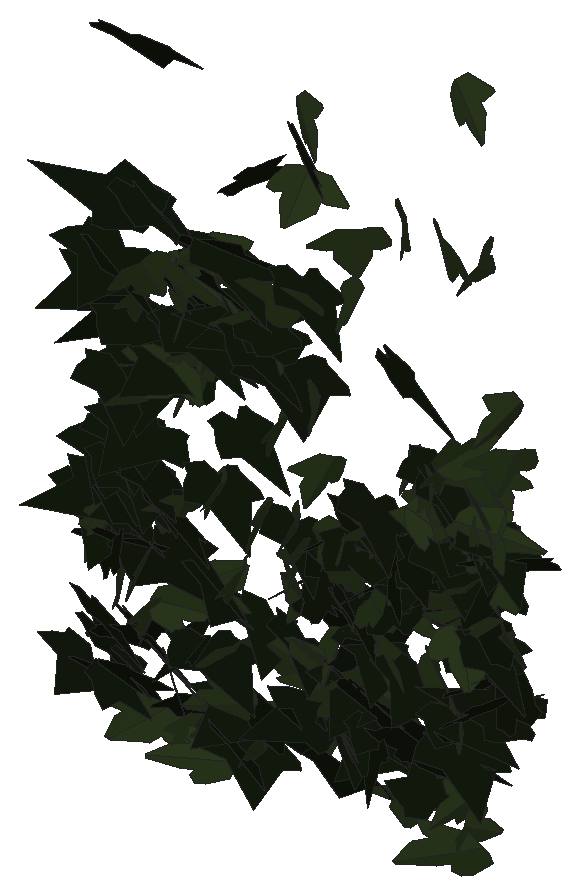
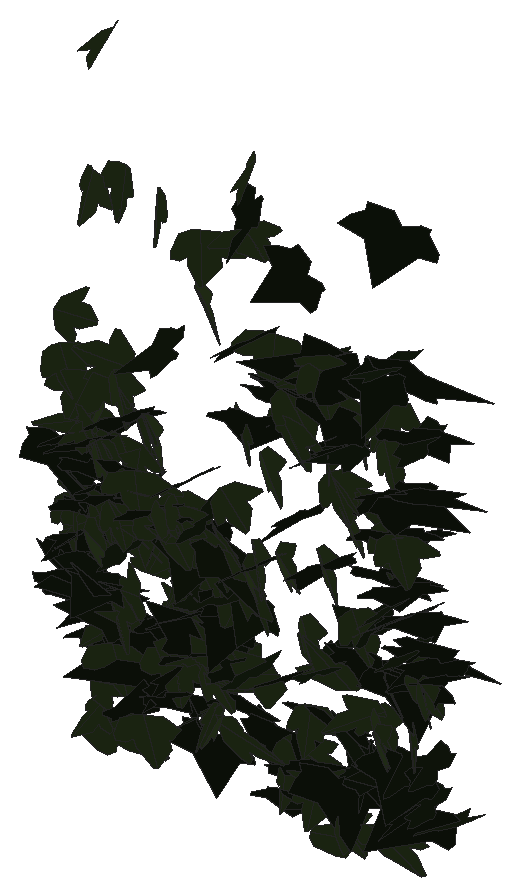
# SketchUp Ruby script. Lengths in millimetres.
U = 1.mm
M = Sketchup.active_model
def pt(a) = Geom::Point3d.new(a.map { |v| v * U })
def face(e, loops, mat)
  f = e.add_face(loops[0].map { |a| pt(a) })
  loops[1..].each { |l| e.add_face(l.map { |a| pt(a) }).erase! }
  f.material = f.back_material = mat if mat
  f
end
# faces: each face lists its corners as indices into pts; further lists are holes
def faces(e, pts, list, mat = nil) = list.each { |f| face(e, (f[0].is_a?(Array) ? f : [f]).map { |l| l.map { |i| pts[i] } }, mat) }
# xy, xz, yz: faces in a plane at the given z, y or x. An outline is a flat list of corners, or four numbers for a rectangle; further outlines are holes
def ring(l) = l.size == 4 ? [[l[0], l[1]], [l[2], l[1]], [l[2], l[3]], [l[0], l[3]]] : l.each_slice(2).to_a
def flat(e, list, mat, &to3) = list.each { |f| face(e, (f[0].is_a?(Array) ? f : [f]).map { |l| ring(l).map { |u, v| to3.(u, v) } }, mat) }
def xy(e, z, list, mat = nil) = flat(e, list, mat) { |x, y| [x, y, z] }
def xz(e, y, list, mat = nil) = flat(e, list, mat) { |x, z| [x, y, z] }
def yz(e, x, list, mat = nil) = flat(e, list, mat) { |y, z| [x, y, z] }
def lines(e, pts, list) = list.each { |a, b| e.add_line(pt(pts[a]), pt(pts[b])) }
# prism: a flat outline (further loops are holes) pulled along v
def prism(e, loops, v, mat = nil)
  f = face(e, loops, mat); d = Geom::Vector3d.new(v.map { |x| x * U })
  f.pushpull(f.normal.samedirection?(d) ? d.length : -d.length)
end
def box(e, o, s, mat = nil) = prism(e, [[o, [o[0] + s[0], o[1], o[2]], [o[0] + s[0], o[1] + s[1], o[2]], [o[0], o[1] + s[1], o[2]]]], [0, 0, s[2]], mat)
def at(x, y, z, deg = 0) = Geom::Transformation.translation(pt([x, y, z])) * Geom::Transformation.rotation(ORIGIN, Z_AXIS, deg.degrees)
def axes(o, x, y, z) = Geom::Transformation.new([*x, 0, *y, 0, *z, 0, *pt(o).to_a, 1])
def part(name) = M.definitions.add(name)
# library, detail: a bought-in or finely detailed component or shape, given as its bounding box
def library(name, o, s) = part(name).tap { |d| box(d.entities, o, s) }
def detail(e, o, s) = box(e.add_group.entities, o, s)
def put(e, d, t, mat = nil) = e.add_instance(d, t).tap { |i| i.material = mat if mat }
def group(e, t, mat = nil) = e.add_group.tap { |g| g.transformation = t; g.material = mat if mat }.entities
root = M.entities
M.materials.add("efeu1").color = [18, 25, 13]
M.materials.add("efeu2").color = [43, 57, 29]
c1 = part("ivyleaf_9")
p = [[39.1,54.8,31.7],[34.5,51.8,30.2],[-5.3,25.2,17.3],[-17.9,28.3,20.9],[-21.6,21.7,17],[-20.2,4.3,5.3],
  [-22.9,-0.3,2.5],[-17.1,-4,-0.6],[-2,-2.1,-1.2],[-0.7,-15.4,-10.1],[16.6,-22.3,-16.7],[21.1,-15.1,-12.5],
  [32.7,-10.7,-11],[46.1,-1.8,-6.6],[30.8,11.2,3.8]]
faces(c1.entities,p,[[0,1,2,3,4,5,6,7,8,9,10,11,12,13,14]],"efeu1")
c2 = part("ivyleaf_10")
p = [[0,12.8,-0.8],[-1.5,51.3,-10.9],[-4.9,51,-11.6],[-13.6,26.5,-7.3],[-13.2,15.9,-4.6],[-21.1,19.3,-7.2],
  [-29.5,16.3,-8.3],[-29.2,8.3,-6.2],[-19.7,-9.8,0.5],[-7.6,-13,4],[1,-12.2,5.8],[-0.4,51.1,-11.1],
  [-1.5,51.1,-10.9],[1,-12.4,5.9],[16.9,-12.4,3.5],[35.1,9.1,-5.1],[35,12.9,-6.1],[20.5,16.4,-4.9],
  [15.8,15,-3.8],[15.3,27.6,-7.1],[12.8,31.3,-7.8]]
faces(c2.entities,p,[[0,1,2,3,4,5,6,7,8,9,10],[11,12,0,13,14,15,16,17,18,19,20]],"efeu2")
put(root,c1,axes([2557.7,915.6,1679.3],[-0.86235,-0.55381,0.54649],[-0.10783,-0.60725,-0.66235],[1.47685,-0.36771,0.27074]))
put(root,c1,axes([2578.8,934.3,2103.4],[-1.36513,-0.35723,0.44081],[-0.65601,-0.29003,-0.79592],[0.85774,-0.79037,0.09283]))
put(root,c1,axes([2557.4,913.3,1886.7],[0.10613,-0.67564,-0.60536],[0.2115,0.60703,-0.66726],[1.71352,-0.03308,0.11986]))
put(root,c2,axes([2575.1,914.1,1848.5],[0.08886,-0.79996,0.47142],[0.28061,-0.45964,-0.79457],[1.74477,0.11466,0.10378]))
put(root,c1,axes([2606.9,906.4,1885.8],[-1.54143,-0.14502,0.48085],[-0.90155,-0.08261,-0.82279],[0.31763,-0.93827,-0.00187]))
put(root,c1,axes([2557.1,925.3,1711.7],[0.82056,-0.74571,0.10087],[0.11253,-0.08233,-0.86132],[1.42774,0.43507,0.00991]))
put(root,c1,axes([2581.2,918.6,1856.9],[-0.7542,-0.79037,0.17718],[-0.09998,-0.17176,-0.88366],[1.53833,-0.39866,0.02944]))
put(root,c2,axes([2589.2,911.8,1862.9],[-0.09793,-0.72878,0.5131],[0.07641,-0.51532,-0.72791],[1.69456,-0.01888,0.06247]))
put(root,c1,axes([2603.4,926.1,2086.3],[-0.25433,0.15373,-0.90287],[0.02132,-0.91209,-0.15696],[-1.74294,-0.03359,0.12983]))
put(root,c1,axes([2626.3,899.9,2221],[-0.73213,0.23685,0.83177],[-1.52357,0.24695,-0.44056],[-0.62282,-0.88252,0.09995]))
put(root,c1,axes([2565.3,910.4,1748],[0.6819,-0.74519,0.28542],[0.26081,-0.25077,-0.82673],[1.49616,0.38335,0.01403]))
put(root,c1,axes([2592.5,919.3,1935.5],[-1.01798,-0.73896,0.00026],[-0.04354,0.01623,-0.91179],[1.40572,-0.53463,-0.02805]))
put(root,c1,axes([2603.4,887.9,1819.2],[0.15333,-0.05162,0.99681],[0.12297,0.99823,0.04647],[-1.89569,0.06058,0.08364]))
put(root,c1,axes([2601,908.6,2162.6],[-1.36967,-0.61543,0.00391],[-0.00564,-0.00255,-0.94693],[1.1713,-0.71967,0.00001]))
put(root,c2,axes([2597.6,910.8,1791.2],[0.54942,-0.77771,-0.35117],[0.0318,0.3758,-0.81852],[1.62372,0.25579,0.13485]))
put(root,c1,axes([2583.8,900.6,1686.7],[1.84357,0.26593,0.01271],[0.02326,0.0035,-1.00451],[-0.50617,0.96875,0.00014]))
put(root,c2,axes([2609.4,920.9,2022.4],[-0.78072,-0.82132,0.04236],[-0.02866,-0.03983,-0.91806],[1.56496,-0.41047,0.00432]))
put(root,c1,axes([2590.7,907.8,1687],[0.53007,-0.62861,-0.64979],[-0.37581,0.62122,-0.6856],[1.67912,0.33748,0.05168]))
put(root,c1,axes([2613.8,897.5,1842.9],[0.99714,0.57705,-0.44003],[-0.75409,-0.22722,-0.76973],[-1.15707,0.64537,0.12244]))
put(root,c1,axes([2604.4,911.9,1735.6],[0.9517,0.74234,0.01204],[0.00712,0.012,-0.89504],[-1.41298,0.50005,0.0036]))
put(root,c1,axes([2583.2,906.3,2154.1],[0.82235,-0.81822,0.1464],[0.16529,-0.11966,-0.92507],[1.57331,0.44024,0.02066]))
put(root,c1,axes([2606,903.6,2026.4],[-0.49833,-0.87659,-0.0428],[0.02692,0.04044,-0.91485],[1.67009,-0.26221,0.00197]))
put(root,c1,axes([2596.1,905.8,1888.3],[0.79963,-0.74213,-0.27037],[-0.16033,0.26239,-0.85114],[1.49467,0.42518,0.05334]))
put(root,c1,axes([2613.3,918.1,1965.3],[-0.70099,-0.83408,-0.11414],[0.06299,0.11014,-0.91168],[1.60098,-0.36954,-0.0141]))
put(root,c1,axes([2602,903.8,1930.6],[0.37398,-0.84872,-0.33656],[0.03436,0.34781,-0.86655],[1.73732,0.17582,0.08959]))
put(root,c2,axes([2636.5,917.8,1645.8],[1.55733,0.0334,-0.48662],[-0.92614,-0.00908,-0.8189],[-0.06347,0.95199,0.00927]))
put(root,c1,axes([2621.6,901.7,2413.2],[1.57535,0.39137,-0.32137],[-0.70697,0.05069,-0.89501],[-0.65507,0.88649,0.19306]))
put(root,c1,axes([2601.6,923.8,1738.7],[1.10253,-0.64432,0.10434],[0.11057,-0.08806,-0.86631],[1.23731,0.582,-0.01556]))
put(root,c1,axes([2606.6,919.1,2089.1],[0.06781,-0.79438,-0.5051],[0.30951,0.50305,-0.77969],[1.76466,-0.05771,0.15616]))
put(root,c2,axes([2631.2,909.8,2128.4],[-0.14476,-0.91791,-0.11043],[0.01893,0.10998,-0.92105],[1.75946,-0.07671,0.00082]))
put(root,c1,axes([2623.5,920.8,2033.4],[-0.91367,-0.79463,-0.12697],[0.14824,0.10127,-0.92828],[1.52433,-0.48614,0.01417]))
put(root,c1,axes([2640.4,912.2,1973.5],[-1.52454,-0.44699,0.04924],[0.00457,-0.10484,-0.91263],[0.85584,-0.79567,0.09258]))
put(root,c2,axes([2631.7,924.2,1766.9],[0.48127,-0.78851,0.29875],[0.22639,-0.27542,-0.82761],[1.58875,0.2781,0.02743]))
put(root,c2,axes([2637.6,901.6,2019.2],[-0.57968,-0.88809,-0.12991],[0.09829,0.11962,-0.93882],[1.70537,-0.30877,0.00995]))
put(root,c1,axes([2627.4,922.9,1916.2],[-0.45803,-0.8481,0.27912],[-0.02478,-0.28571,-0.87937],[1.69908,-0.23279,0.06242]))
put(root,c2,axes([2632.9,902.6,1827.5],[0.63043,-0.76683,0.30919],[0.22263,-0.28626,-0.8353],[1.55777,0.35125,-0.00575]))
put(root,c1,axes([2635.1,912.1,2222.2],[1.38924,-0.05453,-0.60299],[-1.11219,0.18355,-0.72402],[0.30133,0.92883,0.10768]))
put(root,c2,axes([2647.7,903,1781.3],[0.05159,-0.91946,-0.00946],[-0.0071,0.00935,-0.91986],[1.75,0.02714,-0.00346]))
put(root,c1,axes([2629.9,912,1929.7],[0.27736,-0.88683,0.0445],[0.007,-0.04449,-0.89871],[1.68991,0.14573,-0.00358]))
put(root,c2,axes([2646.3,886.4,2167.5],[-0.6468,-0.76653,-0.47902],[0.41332,0.42753,-0.83821],[1.66991,-0.40271,0.02193]))
put(root,c1,axes([2626,903,2239.1],[0.8863,-0.80954,-0.25065],[0.15642,0.32779,-0.906],[1.60527,0.41502,0.22667]))
put(root,c2,axes([2668,903.4,2055.2],[1.64546,-0.23184,-0.3469],[-0.64243,0.0805,-0.89507],[0.46676,0.92809,-0.00902]))
put(root,c1,axes([2677.2,915.6,2055.3],[-1.46751,-0.41641,0.31827],[-0.13036,-0.48124,-0.79559],[0.98894,-0.68136,0.36741]))
put(root,c2,axes([2673.2,913.3,1899.8],[-0.53716,-0.88714,0.06992],[-0.04075,-0.06656,-0.93095],[1.69315,-0.28305,-0.00023]))
put(root,c2,axes([2661.2,905.9,1783.7],[0.19263,0.31723,0.83976],[0.35443,0.81928,-0.33193],[-1.6713,0.2103,0.02639]))
put(root,c2,axes([2677.1,928,1645.7],[-0.04551,-0.7945,0.37788],[0.09886,-0.37864,-0.7928],[1.6715,0.00076,0.05718]))
put(root,c2,axes([2677.4,925.4,2037],[0.60301,-0.86275,0.11117],[0.05097,-0.10858,-0.91901],[1.65478,0.31773,-0.0122]))
put(root,c1,axes([2684.8,883.1,1721.2],[0.75081,-0.20496,-0.81986],[-1.38164,0.381,-0.44457],[0.82337,0.82622,0.00162]))
put(root,c1,axes([2652.4,911.4,1715.1],[1.14728,-0.23133,-0.64445],[1.11081,-0.27534,0.64479],[-0.68138,-0.83838,-0.03394]))
put(root,c1,axes([2648.2,904.7,1846.7],[-0.03954,-0.44661,-0.91834],[1.37818,0.6412,-0.32821],[1.37034,-0.65776,0.30359]))
put(root,c1,axes([2658.8,911.1,1890.1],[0.23979,-0.76384,0.51831],[0.48694,-0.47373,-0.76032],[1.688,0.24516,0.1457]))
put(root,c1,axes([2661.2,922.7,2133.9],[1.2412,-0.66483,-0.05791],[-0.0515,0.05456,-0.9311],[1.26904,0.65245,0.01886]))
put(root,c1,axes([2697.1,913.4,1755.6],[-1.11964,0.48867,-0.44066],[0.61544,-0.30009,-0.76449],[-1.09067,-0.67098,0.02098]))
put(root,c2,axes([2709.6,920.5,1617.7],[-0.33286,0.14893,0.82216],[-0.97452,-0.68287,0.01478],[1.2566,-0.49013,0.22924]))
put(root,c2,axes([2691.1,888.6,2137.7],[0.67195,-0.79138,-0.35145],[-0.07911,0.36362,-0.86053],[1.6461,0.34052,0.10211]))
put(root,c2,axes([2693.6,925.8,2074.1],[-0.41972,-0.89404,0.11918],[-0.00102,-0.12256,-0.92039],[1.71659,-0.21867,0.02859]))
put(root,c1,axes([2700,912.9,1687.4],[0.60838,0.86572,-0.27736],[-0.19769,-0.25729,-0.92282],[-1.71881,0.33602,0.00797]))
put(root,c2,axes([2673.3,914.1,2163.7],[-0.63802,0.05692,-0.8855],[1.40617,-0.5063,-0.31226],[-0.93521,-0.8001,0.13461]))
put(root,c2,axes([2697.9,917.8,2069.5],[1.1316,-0.67331,0.27501],[0.30794,-0.22385,-0.89789],[1.34953,0.61566,-0.02571]))
put(root,c1,axes([2683.4,905.1,2117.3],[0.53656,-0.74172,-0.53908],[0.17927,0.58443,-0.75485],[1.73586,0.16891,0.24459]))
put(root,c2,axes([2712.6,913.9,2091.7],[0.42986,-0.89414,-0.1785],[0.26236,0.21527,-0.90389],[1.71535,0.19114,0.18298]))
put(root,c1,axes([2698.6,897.8,2120.5],[0.24929,-0.87528,-0.38354],[0.1294,0.39468,-0.87749],[1.81414,0.09212,0.1153]))
put(root,c2,axes([2724.3,914.4,2197.3],[-0.79361,-0.84809,0.02305],[0.00425,-0.02678,-0.94495],[1.61467,-0.41676,0.01382]))
put(root,c1,axes([2684.9,913,2156.2],[0.6677,0.07038,-0.88332],[1.65633,0.15141,0.35772],[0.31736,-0.9383,-0.00853]))
put(root,c2,axes([2699.4,913.3,1818.3],[1.36333,-0.20374,-0.56691],[1.02678,-0.1749,0.74456],[-0.51007,-0.89662,-0.01642]))
put(root,c2,axes([2726.3,918.3,1669.1],[-0.67872,-0.73111,-0.3171],[0.25756,0.2868,-0.81344],[1.49467,-0.38142,-0.00382]))
put(root,c2,axes([2734.5,895.4,1948.5],[0.38047,-0.88318,-0.08378],[-0.01598,0.08399,-0.90547],[1.68835,0.19982,0.01031]))
put(root,c2,axes([2761.3,908.8,1705.5],[-0.85514,-0.21321,0.78121],[-1.35187,-0.32525,-0.4973],[0.74007,-0.84047,-0.00573]))
put(root,c1,axes([2725.7,916,1818.9],[-0.50527,-0.5929,0.6501],[0.04186,-0.68331,-0.61421],[1.67403,-0.16187,0.21158]))
put(root,c2,axes([2713.5,905.3,2202],[-0.78904,-0.40408,-0.76936],[1.32735,0.35383,-0.56166],[0.9867,-0.79912,0.14033]))
put(root,c1,axes([2715.3,906.8,1757.6],[-0.61435,-0.48529,-0.66571],[1.18967,0.32144,-0.53742],[1.02127,-0.66637,0.22558]))
put(root,c2,axes([2739.9,912.1,1756.4],[-0.64268,-0.77554,-0.29308],[0.22192,0.26888,-0.84587],[1.56219,-0.35725,-0.00041]))
put(root,c1,axes([2702.7,906.3,2197.4],[1.30198,-0.05676,0.67383],[1.28577,0.09884,-0.67756],[-0.05568,0.95513,0.11016]))
put(root,c1,axes([2727.7,905.8,1949.5],[0.00574,-0.9132,-0.26924],[-0.06795,0.26895,-0.9126],[1.8107,0.01299,-0.0334]))
put(root,c1,axes([2757.2,922.3,1691.6],[-1.30833,-0.50128,0.24516],[-0.35332,-0.16139,-0.85055],[1.00153,-0.71178,0.0202]))
put(root,c2,axes([2757.1,898.3,1854.9],[0.16699,-0.89879,-0.16351],[-0.02093,0.16321,-0.90305],[1.73852,0.0883,0.00483]))
put(root,c1,axes([2737.4,906.6,2207.9],[-0.00837,-0.94535,0.05301],[0.45093,-0.05243,-0.91523],[1.74469,0.00902,0.2368]))
put(root,c1,axes([2738.3,912.7,1655.9],[0.175,-0.65032,0.53623],[0.40225,-0.50439,-0.64795],[1.55293,0.20393,0.10741]))
put(root,c1,axes([2746.4,913.1,2014.2],[0.42839,-0.76528,-0.46033],[-0.14691,0.45628,-0.79629],[1.69332,0.23319,0.04737]))
put(root,c2,axes([2771.9,906.6,2144.2],[-0.60951,-0.86998,0.20243],[-0.1708,-0.18262,-0.92683],[1.69138,-0.33195,-0.02065]))
put(root,c2,axes([2767.2,917.9,2118.1],[1.5021,-0.47005,-0.20203],[-0.26847,0.15709,-0.91657],[0.93598,0.79941,0.06132]))
put(root,c1,axes([2758.2,921.4,1655.7],[-0.91145,-0.67172,-0.25991],[0.37808,0.17682,-0.82303],[1.31761,-0.5154,0.05637]))
put(root,c1,axes([2761.3,896.6,2301.8],[0.68712,0.55969,0.69828],[0.76449,0.57149,-0.66576],[-1.52196,0.53975,-0.01917]))
put(root,c1,axes([2808.7,901.7,2151.2],[-1.48294,0.34542,0.40853],[-0.89681,-0.10136,-0.81303],[-0.48212,-0.87393,0.25577]))
put(root,c2,axes([2777,907.7,1671],[-0.08853,-0.72628,-0.52307],[0.11345,0.5201,-0.72746],[1.69964,-0.07255,0.02131]))
put(root,c1,axes([2802.4,907.1,2147.4],[-1.64736,-0.19065,0.32604],[-0.59899,-0.08657,-0.88618],[0.39736,-0.92088,0.01581]))
put(root,c1,axes([2775.7,929.2,1797.3],[-0.50733,-0.81591,0.24377],[-0.03684,-0.24957,-0.85646],[1.62024,-0.26115,0.05686]))
put(root,c2,axes([2785,904,1934.8],[0.47845,-0.80054,0.33629],[0.21423,-0.3171,-0.83901],[1.63862,0.2752,0.0115]))
put(root,c1,axes([2768.4,900.9,2129.8],[0.5445,-0.8721,-0.29312],[-0.04375,0.30009,-0.91528],[1.75047,0.27877,0.0683]))
put(root,c1,axes([2812.1,898.4,1687.9],[0.13018,-0.1847,0.92206],[-0.89061,0.79522,0.19401],[-1.5524,-0.4717,-0.03398]))
put(root,c2,axes([2810.8,891.3,2193.7],[-1.74215,-0.25601,0.01241],[-0.03645,0.02243,-0.95013],[0.48645,-0.91519,-0.02676]))
put(root,c2,axes([2810.3,901.7,2047],[0.31257,-0.91899,-0.00136],[0.01066,0.00238,-0.93354],[1.749,0.16422,0.00593]))
put(root,c2,axes([2848.7,917.7,1699.1],[0.09979,0.20816,0.87879],[-1.70947,0.10359,0.02905],[-0.17881,-0.87424,0.21269]))
put(root,c2,axes([2820.9,906.3,1932.7],[0.34984,-0.86777,-0.30896],[0.02253,0.31725,-0.88402],[1.75296,0.16911,0.07302]))
put(root,c2,axes([2836.5,889.6,1861.6],[0.17509,-0.22957,-0.878],[-0.59587,0.82029,-0.24729],[1.62114,0.3263,0.00394]))
put(root,c1,axes([2817.1,912.3,2106.7],[-1.07471,-0.64212,-0.4449],[0.60873,0.3108,-0.85453],[1.35643,-0.64824,0.03099]))
put(root,c1,axes([2829.8,900.4,1867.6],[0.41934,0.76144,0.49287],[0.20508,0.48164,-0.79226],[-1.71405,0.24391,0.02579]))
put(root,c1,axes([2815.2,928.5,1787.2],[-0.13196,-0.77836,0.50808],[0.05826,-0.51112,-0.77885],[1.76807,-0.04125,0.06358]))
put(root,c1,axes([2816.9,918.6,1922.1],[-0.0831,-0.90714,0.04068],[-0.01293,-0.0404,-0.90818],[1.72816,-0.04393,-0.00484]))
put(root,c2,axes([2829.5,907.5,1905.1],[0.47337,-0.77204,0.41701],[0.34407,-0.37906,-0.80959],[1.63416,0.30345,0.04966]))
put(root,c1,axes([2857.6,897.3,1728],[-1.61088,0.15478,0.08343],[-0.16127,0.00032,-0.86031],[-0.29321,-0.85051,0.01485]))
put(root,c2,axes([2835.7,919,1883.4],[-1.66137,0.16843,-0.07553],[0.14749,0.00302,-0.88886],[-0.31887,-0.87619,-0.01758]))
put(root,c1,axes([2837.4,894.2,2366.9],[1.08927,-0.31792,-0.72658],[-1.18126,0.37824,-0.65441],[0.93964,0.84405,0.01959]))
put(root,c2,axes([2814.1,907.1,1781.3],[-0.95604,0.10722,-0.7816],[1.47384,-0.10996,-0.51279],[-0.28676,-0.92258,-0.02972]))
put(root,c2,axes([2841.8,898.8,2328.6],[1.02056,0.70675,-0.40833],[-0.4249,-0.34294,-0.88675],[-1.49422,0.58024,-0.02673]))
put(root,c1,axes([2828,913,2203.2],[0.20958,-0.92285,-0.20654],[-0.02239,0.20658,-0.92932],[1.79969,0.11004,0.01249]))
put(root,c2,axes([2842.6,895,2409.2],[-0.36484,0.96324,-0.01831],[-0.11976,-0.03114,-0.97979],[-1.82966,-0.19003,0.06778]))
put(root,c2,axes([2849.9,922,1999.4],[-0.38945,-0.8275,0.37986],[0.08795,-0.39827,-0.84272],[1.73068,-0.16597,0.1283]))
put(root,c1,axes([2864.8,920.5,1925.8],[-0.35695,0.80911,-0.30417],[0.02006,-0.30909,-0.82868],[-1.645,-0.17934,0.0559]))
put(root,c2,axes([2871,909.8,1765.4],[-1.48508,-0.24032,-0.53592],[-0.97648,-0.15483,0.81647],[-0.54406,0.93387,-0.00254]))
put(root,c2,axes([2854.1,893.7,2085.8],[0.77085,-0.7941,-0.26058],[-0.03615,0.28075,-0.88508],[1.5902,0.39132,0.10619]))
put(root,c1,axes([2851.7,917,1843.2],[1.39678,-0.03562,-0.48159],[-0.91508,0.02773,-0.73476],[0.08563,0.87738,0.00367]))
put(root,c1,axes([2864.4,904.4,1850.4],[0.45009,0.58446,0.62609],[-1.222,-0.30889,0.53088],[1.07882,-0.59372,0.34013]))
put(root,c2,axes([2873.2,916.3,1913.9],[-1.55371,0.30529,0.21632],[-0.44255,-0.00721,-0.86737],[-0.55789,-0.84451,0.0856]))
put(root,c2,axes([2889.4,897.7,1911.5],[-1.13617,0.32987,0.60549],[-1.11705,0.1772,-0.67522],[-0.6887,-0.83162,0.0963]))
put(root,c2,axes([2871.4,907.1,1934.8],[1.00953,-0.7408,-0.01632],[-0.01781,0.01337,-0.91112],[1.41012,0.53052,0.00017]))
put(root,c2,axes([2878.7,911.2,1761.6],[-0.20185,-0.89547,0.25789],[-0.00785,-0.2591,-0.90138],[1.77352,-0.10306,0.02536]))
put(root,c1,axes([2878.7,907.1,1678.4],[1.21836,0.26012,-0.52154],[-0.94354,-0.16425,-0.69044],[-0.58315,0.80922,0.0275]))
put(root,c2,axes([2873.4,913.9,1711.4],[-0.86318,0.78711,-0.00919],[0.00207,-0.00998,-0.90842],[-1.49813,-0.45352,0.00404]))
put(root,c1,axes([2866.3,935.2,1867.2],[-0.44044,-0.75339,0.43693],[0.41596,-0.48787,-0.72545],[1.6045,-0.08033,0.30801]))
put(root,c2,axes([2883.9,911,1711.9],[-0.5485,0.74799,0.43423],[-0.35053,0.39413,-0.80115],[-1.60832,-0.341,0.02652]))
put(root,c2,axes([2874.5,904.1,1819.2],[0.82189,-0.69209,0.40773],[0.40722,-0.34708,-0.81577],[1.47355,0.48194,-0.00198]))
put(root,c1,axes([2859.4,910.7,1781.7],[0.93399,-0.58891,0.47638],[0.66814,-0.32615,-0.76484],[1.27743,0.60117,0.05173]))
put(root,c1,axes([2883,923.6,1714.7],[-0.15636,-0.82556,0.30845],[-0.07878,-0.30583,-0.82957],[1.67544,-0.09142,-0.01022]))
put(root,c2,axes([2919.9,919.4,1784.7],[1.10363,0.04419,-0.70175],[-1.33569,0.09223,-0.57413],[0.08217,0.90566,0.09271]))
put(root,c2,axes([2905.3,896.2,2222.5],[0.72132,-0.88542,-0.04677],[-0.03093,0.04392,-0.96312],[1.68719,0.37934,0.00234]))
put(root,c1,axes([2908.1,916.8,1772.5],[-1.14592,-0.62334,0.08925],[-0.11084,-0.06783,-0.86663],[1.1933,-0.60489,0.00521]))
put(root,c2,axes([2931.7,917.6,1942.6],[0.81001,0.09275,-0.80304],[-1.53152,0.13493,-0.41091],[0.14634,0.89878,0.14455]))
put(root,c2,axes([2910,893.7,2290.6],[-1.0208,-0.82147,-0.06115],[0.17031,0.01443,-0.97878],[1.55847,-0.53964,0.06691]))
put(root,c1,axes([2884.3,921,1956.7],[0.63486,-0.84112,0.18283],[0.13957,-0.16759,-0.90483],[1.63224,0.34148,0.00626]))
put(root,c1,axes([2893.2,910.7,1855.9],[0.23009,-0.66184,0.61024],[0.14364,-0.6061,-0.6723],[1.70729,0.14019,-0.02568]))
put(root,c1,axes([2901.2,911.5,1795.8],[-0.15828,-0.27642,0.86094],[1.45033,0.44397,0.21616],[-0.92636,0.74232,0.19131]))
put(root,c1,axes([2920.9,899.9,1894.6],[0.36889,0.78185,0.38972],[0.21647,0.37321,-0.8053],[-1.64848,0.22397,-0.01854]))
put(root,c2,axes([2923.9,913.5,1959.6],[-0.33148,-0.89754,0.09825],[-0.05432,-0.09454,-0.91423],[1.71754,-0.17621,-0.00995]))
put(root,c2,axes([2933.5,915.6,1759.3],[-1.6294,0.15785,0.30309],[-0.57105,0.04409,-0.87051],[-0.31129,-0.90713,0.01043]))
put(root,c1,axes([2932.4,924.3,1716.8],[-1.28725,-0.5024,0.20746],[-0.29093,-0.142,-0.84225],[0.99274,-0.69307,0.02218]))
put(root,c1,axes([2905.2,908.2,1939.4],[-0.18354,-0.71579,-0.59865],[0.27147,0.58346,-0.7206],[1.75507,-0.1651,0.04886]))
put(root,c2,axes([2943.9,920.2,1934.2],[-1.52917,-0.04527,0.45626],[-0.85809,-0.08926,-0.80284],[0.15856,-0.91966,0.05546]))
put(root,c1,axes([2919.4,922.6,1821.4],[-0.56932,-0.82493,0.19051],[-0.03586,-0.19552,-0.87618],[1.61092,-0.29589,0.04783]))
put(root,c2,axes([2922,904.2,1876.6],[-0.1269,-0.76893,-0.42899],[0.50484,0.39269,-0.7451],[1.59793,-0.18513,0.20133]))
put(root,c1,axes([2919.3,909.1,1719],[-0.80072,0.13063,-0.75248],[1.32103,-0.29297,-0.43895],[-0.60634,-0.8108,0.03738]))
put(root,c2,axes([2935.4,926.4,1955.3],[-0.14613,-0.81983,0.38889],[-0.03649,-0.38872,-0.82327],[1.72655,-0.0776,0.01552]))
put(root,c1,axes([2921.9,907.7,1744.4],[0.20714,-0.57616,-0.64225],[-0.25618,0.62808,-0.58625],[1.622,0.17278,-0.01057]))
put(root,c1,axes([2922.6,907.6,1988.7],[-0.08428,-0.92209,0.0919],[-0.02423,-0.09139,-0.92311],[1.76344,-0.04532,-0.00829]))
put(root,c2,axes([2914.4,909.6,1823.9],[1.09752,-0.23355,0.67278],[1.25334,-0.15469,-0.61816],[0.51599,0.8725,0.07049]))
put(root,c1,axes([2950.2,902.7,1865.9],[-1.21961,0.64069,-0.17112],[-0.29057,0.08903,0.90508],[1.22819,0.65727,0.0442]))
put(root,c2,axes([2935.6,920.9,1912.7],[1.60174,0.13114,0.2751],[0.42455,0.28542,-0.8185],[-0.39519,0.83816,0.23568]))
put(root,c1,axes([2919.2,903.8,1752.1],[0.13808,-0.40244,1.01679],[1.40801,-0.73236,-0.34266],[1.53264,0.70907,0.22319]))
put(root,c2,axes([2966.7,921.4,1668.2],[-1.30308,-0.53058,0.13792],[-0.193,-0.09429,-0.86611],[1.02535,-0.69204,0.01226]))
put(root,c1,axes([2956.3,924.3,1946.2],[-0.73304,-0.83459,-0.0298],[0.02414,0.02697,-0.91918],[1.58922,-0.38537,0.00022]))
put(root,c1,axes([2964.4,883.8,1928.4],[0.58638,-0.25107,-0.81837],[-1.14421,0.55569,-0.39683],[1.15975,0.67519,0.02227]))
put(root,c1,axes([2940.6,911.5,2152],[1.17385,-0.73433,-0.17989],[-0.20555,0.1442,-0.95893],[1.42414,0.62608,0.00987]))
put(root,c2,axes([2968.2,913.6,2045.8],[0.464,-0.87203,-0.24082],[-0.15387,0.22741,-0.90533],[1.71488,0.25635,-0.01607]))
put(root,c2,axes([2965.1,897.5,2325.6],[0.69303,-0.78088,-0.4151],[0.19154,0.48258,-0.81955],[1.67216,0.26836,0.26591]))
put(root,c1,axes([2970.4,917.3,1800.8],[-0.63512,-0.69729,0.46265],[-0.17475,-0.46456,-0.76641],[1.58302,-0.33105,0.10102]))
put(root,c2,axes([2976.4,928.1,1979.2],[-1.38616,-0.53396,0.11151],[0.13624,-0.27797,-0.86349],[1.02917,-0.68237,0.26449]))
put(root,c2,axes([2950.6,915.4,1882],[-0.47071,-0.03994,0.91667],[1.72821,0.12549,0.25047],[-0.25041,0.94112,0.0055]))
put(root,c1,axes([2994.5,909.9,1672.2],[-1.00108,-0.50541,0.58798],[0.80022,0.41104,0.72945],[-1.23982,0.67339,-0.00395]))
put(root,c2,axes([2981.1,904.3,1996.1],[0.02315,0.69272,0.62534],[0.06818,0.62458,-0.69259],[-1.77481,0.03303,-0.01845]))
put(root,c2,axes([2991.1,900.9,2039.7],[0.96237,-0.74084,-0.2527],[-0.09432,0.26994,-0.89055],[1.48675,0.49667,0.10708]))
put(root,c1,axes([2984.1,881.7,1958.2],[0.93601,-0.18705,-0.77102],[-0.86643,0.6764,-0.45448],[1.23664,0.61549,0.26515]))
put(root,c1,axes([2957.3,904.9,1722.8],[0.41071,-0.27569,0.81243],[1.48167,-0.28908,-0.30489],[0.68609,0.78933,0.17209]))
put(root,c2,axes([3001.1,910.7,2006.8],[1.49393,-0.42416,-0.25464],[-0.27763,0.2579,-0.87927],[0.89971,0.78389,0.15149]))
put(root,c1,axes([2968,907.2,1742.4],[1.74533,0.06919,0.33829],[0.64324,0.01671,-0.91962],[-0.13456,0.97732,-0.00823]))
put(root,c2,axes([3005,922.9,1930.6],[-0.48528,-0.87423,0.02858],[0.0808,-0.04211,-0.90914],[1.66277,-0.2531,0.05252]))
put(root,c2,axes([3013.6,917.8,1740.3],[-1.40991,-0.38851,0.17924],[-0.27239,-0.11272,-0.83587],[0.76741,-0.7538,0.03261]))
put(root,c1,axes([3032.4,922.9,1942.8],[-1.50517,-0.15544,0.42751],[-0.74538,-0.20346,-0.7985],[0.44037,-0.87569,0.10964]))
put(root,c1,axes([2988.4,930.9,1886.1],[0.5387,-0.83105,0.13109],[0.10627,-0.11945,-0.87782],[1.59768,0.28815,0.01419]))
put(root,c1,axes([3000.6,922,2048.9],[-0.40888,-0.9064,-0.06104],[-0.00242,0.06302,-0.93138],[1.72897,-0.21427,-0.01574]))
put(root,c2,axes([3036.2,905.8,1637.8],[-0.79048,-0.28419,0.85261],[-1.11057,-0.62908,-0.49394],[1.30088,-0.70973,0.09641]))
put(root,c2,axes([2984.9,914.6,1824.5],[0.45371,-0.32064,0.81146],[1.35774,-0.41267,-0.37265],[0.95604,0.73824,0.14413]))
put(root,c1,axes([3002.8,921.1,2034.5],[0.13126,-0.93395,0.015],[-0.04158,-0.01665,-0.93621],[1.77724,0.06859,-0.02301]))
put(root,c2,axes([3027,898.4,1788.3],[0.874,-0.45406,-0.66565],[-0.41951,0.66614,-0.60647],[1.47503,0.4585,0.22193]))
put(root,c2,axes([3023.7,896.8,2073.5],[-0.04155,-0.91782,-0.19191],[-0.01242,0.19211,-0.91801],[1.78452,-0.02003,-0.01086]))
put(root,c2,axes([3026.1,924.6,1995.5],[0.03055,-0.91915,-0.05234],[-0.05067,0.05186,-0.91893],[1.75142,0.01753,-0.02567]))
put(root,c2,axes([3032.7,883.7,2327.9],[-1.20988,0.65895,0.3624],[-0.5487,0.22473,-0.91436],[-1.32191,-0.69639,0.04785]))
put(root,c1,axes([3013,921.3,1960.3],[-0.35938,-0.89614,-0.10866],[0.07782,0.10241,-0.91563],[1.71627,-0.19229,0.01876]))
put(root,c1,axes([3034.1,936.4,1984.3],[-1.43311,-0.51193,0.01515],[-0.0159,-0.01465,-0.91051],[0.97461,-0.75301,0.00742]))
put(root,c2,axes([3033.3,905.7,1927.6],[-0.49298,-0.88105,-0.13872],[0.0646,0.13461,-0.91832],[1.69624,-0.26118,-0.00534]))
put(root,c2,axes([3035.8,911.7,1694.1],[-0.10096,-0.36828,0.84343],[0.12337,-0.84423,-0.36455],[1.74722,0.03833,0.07448]))
put(root,c1,axes([3073.5,905.5,1893.3],[-0.89146,-0.04706,-0.80742],[-1.42476,-0.32794,0.4534],[-0.58262,0.87395,0.12666]))
put(root,c2,axes([3020.9,900.1,1772.6],[0.56832,0.64093,0.53578],[0.47867,0.47361,-0.70673],[-1.51612,0.38978,-0.02229]))
put(root,c2,axes([3031.9,935.3,1893.1],[0.45166,-0.66291,0.5677],[0.39886,-0.52782,-0.70395],[1.61247,0.31625,0.01511]))
put(root,c1,axes([3041.8,936.6,1934.3],[-1.02689,-0.73118,0.03863],[-0.03293,-0.03523,-0.90868],[1.39313,-0.53979,0.00699]))
put(root,c1,axes([3027.4,898.2,1778.9],[0.74133,0.07196,0.79449],[0.92695,0.67878,-0.30027],[-1.20246,0.56763,0.25835]))
put(root,c2,axes([3038.8,910.9,1662.6],[-0.15883,-0.44258,-0.76989],[0.50313,0.72584,-0.44592],[1.61348,-0.26991,0.06326]))
put(root,c2,axes([3057.1,901.6,1904.1],[-1.36398,-0.53487,0.18646],[-0.29344,-0.10514,-0.89423],[1.03734,-0.73304,-0.00779]))
put(root,c1,axes([3030.3,895.6,1798.1],[0.19333,-0.50291,-0.73544],[0.08901,0.74219,-0.50107],[1.69331,0.0184,0.11031]))
put(root,c1,axes([3043.9,893,1910.9],[-0.72649,0.85567,0.03737],[0.01955,-0.03634,0.93694],[1.62995,0.38182,0.00542]))
put(root,c1,axes([3046.5,901.2,1826.1],[0.71603,0.72103,0.35586],[0.29213,0.32126,-0.8132],[-1.50216,0.40617,0.01148]))
put(root,c1,axes([3038.7,900,1759],[-0.41901,-0.88269,-0.2571],[0.11147,0.25037,-0.90972],[1.74619,-0.22779,-0.00362]))
put(root,c2,axes([3041.1,880.8,2086.3],[-0.13951,-0.57656,0.80241],[0.14662,0.79883,0.58102],[-1.87476,0.10538,-0.01427]))
put(root,c2,axes([3047.8,924.1,1937.2],[1.60656,-0.30051,-0.03469],[-0.06074,0.01379,-0.89603],[0.57252,0.84473,0.00229]))
put(root,c2,axes([3043,895.7,1881.8],[1.08344,0.81098,-0.01658],[-0.02157,-0.0123,-0.99084],[-1.54363,0.56938,0.00221]))
put(root,c2,axes([3049.8,888.4,2504.7],[-0.03821,0.99355,0.08252],[0.01101,0.08265,-0.99372],[-1.8974,-0.01953,-0.00743]))
put(root,c2,axes([3068.5,913.7,2024.7],[0.78198,-0.60071,-0.54336],[-0.58133,0.44938,-0.72778],[1.42777,0.51197,0.00127]))
put(root,c2,axes([3051.2,903.1,2039.1],[-0.80127,0.8124,-0.10164],[0.12553,-0.08027,-0.91476],[-1.55315,-0.42561,-0.0215]))
put(root,c2,axes([3064.1,893.6,2314.2],[-0.18836,-0.6513,-0.78315],[0.13085,0.78077,-0.65801],[1.93414,-0.11625,-0.03175]))
put(root,c1,axes([3055.9,928.4,1999.5],[-0.58026,-0.86682,0.09621],[0.01925,-0.10542,-0.91781],[1.65975,-0.30182,0.04428]))
put(root,c2,axes([3059.6,909.7,2067.1],[-1.45328,-0.49705,-0.23383],[0.47529,0.04252,-0.90589],[0.93115,-0.79746,0.09744]))
put(root,c2,axes([3060.8,910.1,2013],[0.23349,0.89001,-0.16681],[-0.22758,-0.15093,-0.89326],[-1.70827,0.14176,0.0962]))
put(root,c1,axes([3095.7,919.8,1800.7],[-0.71279,0.04394,0.80373],[-1.51618,-0.14707,-0.36318],[0.21919,-0.87443,0.10147]))
put(root,c2,axes([3067.8,904.4,1999.2],[1.29111,-0.57257,-0.16024],[-0.18614,0.13233,-0.88693],[1.11617,0.68438,0.03744]))
put(root,c1,axes([3048.3,912.2,1875.3],[-0.0491,-0.68991,-0.5944],[0.40174,0.57391,-0.6753],[1.68595,-0.15685,0.1436]))
put(root,c1,axes([3099.6,904.2,1812.4],[-0.18262,0.22694,0.95168],[-0.77094,0.86122,-0.24621],[-1.69493,-0.41618,0.00945]))
put(root,c1,axes([3059.7,891.4,1806.5],[0.7901,0.27726,0.73871],[0.85901,0.60122,-0.4793],[-1.23173,0.59714,0.13958]))
put(root,c2,axes([3091.9,904.1,1899.9],[-0.94423,0.42686,0.67185],[-0.96265,0.44222,-0.65447],[-1.16973,-0.7085,-0.00372]))
put(root,c1,axes([3059.3,909.3,1879.2],[0.37586,-0.84521,-0.21545],[-0.07639,0.21186,-0.86793],[1.65829,0.20133,0.00885]))
put(root,c1,axes([3088.8,911,1979.7],[0.5283,0.82426,-0.3033],[-0.38978,-0.24858,-0.86297],[-1.62548,0.3275,0.10836]))
put(root,c1,axes([3067.6,916.6,2003.1],[-0.12849,-0.91605,-0.14778],[0.06214,0.14574,-0.91828],[1.76488,-0.07183,0.02157]))
put(root,c2,axes([3055.3,895.3,2015.6],[-0.54389,-0.27746,-0.85204],[1.5198,0.32687,-0.37428],[0.7737,-0.83713,0.13625]))
put(root,c2,axes([3087.7,915.1,2094.3],[-0.76956,-0.84929,0.10834],[0.02628,-0.12627,-0.9383],[1.62926,-0.39911,0.06631]))
put(root,c2,axes([3086,914.3,2148.3],[-0.03504,-0.48837,0.86162],[0.22539,-0.85667,-0.48304],[1.87141,0.09403,0.07431]))
